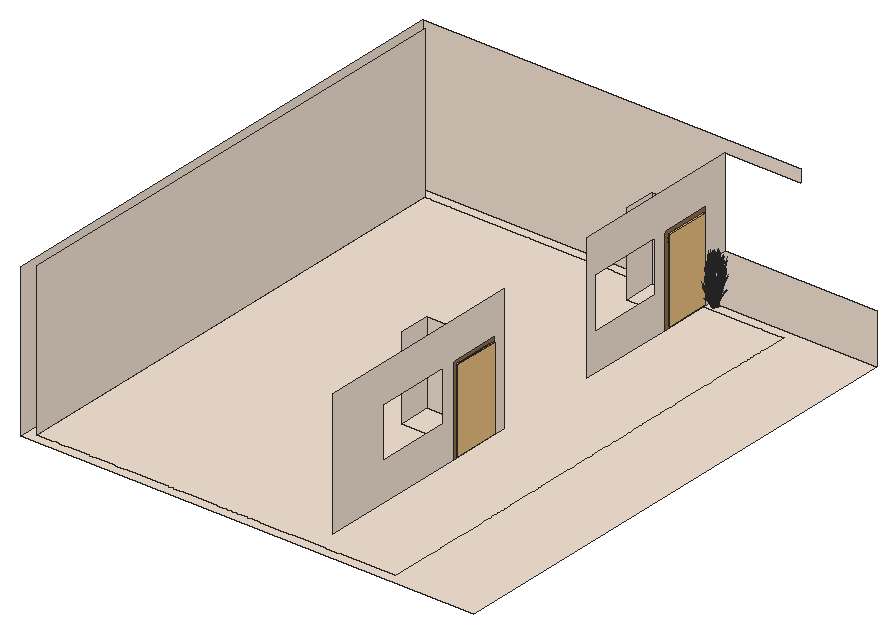
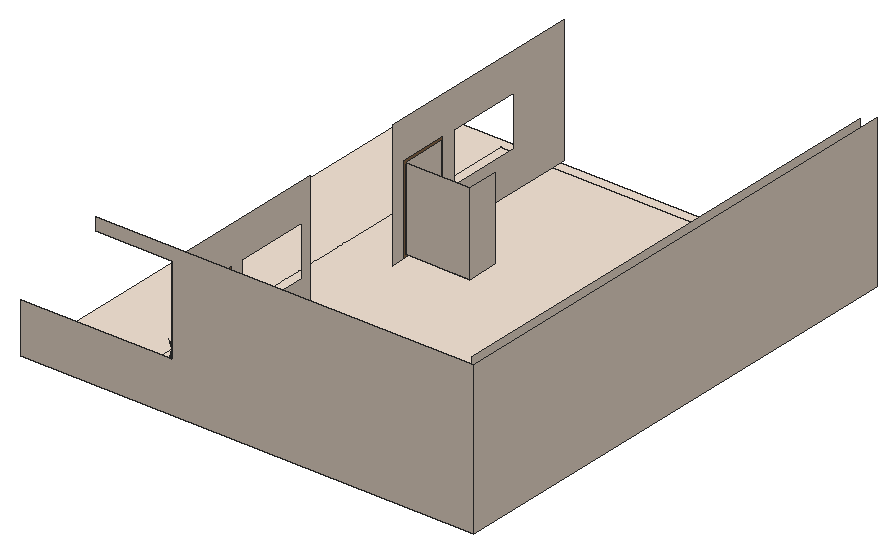
# SketchUp Ruby script. Lengths in inches.
U = 1.inch
M = Sketchup.active_model
def pt(a) = Geom::Point3d.new(a.map { |v| v * U })
def face(e, loops, mat)
  f = e.add_face(loops[0].map { |a| pt(a) })
  loops[1..].each { |l| e.add_face(l.map { |a| pt(a) }).erase! }
  f.material = f.back_material = mat if mat
  f
end
# faces: each face lists its corners as indices into pts; further lists are holes
def faces(e, pts, list, mat = nil) = list.each { |f| face(e, (f[0].is_a?(Array) ? f : [f]).map { |l| l.map { |i| pts[i] } }, mat) }
# xy, xz, yz: faces in a plane at the given z, y or x. An outline is a flat list of corners, or four numbers for a rectangle; further outlines are holes
def ring(l) = l.size == 4 ? [[l[0], l[1]], [l[2], l[1]], [l[2], l[3]], [l[0], l[3]]] : l.each_slice(2).to_a
def flat(e, list, mat, &to3) = list.each { |f| face(e, (f[0].is_a?(Array) ? f : [f]).map { |l| ring(l).map { |u, v| to3.(u, v) } }, mat) }
def xy(e, z, list, mat = nil) = flat(e, list, mat) { |x, y| [x, y, z] }
def xz(e, y, list, mat = nil) = flat(e, list, mat) { |x, z| [x, y, z] }
def yz(e, x, list, mat = nil) = flat(e, list, mat) { |y, z| [x, y, z] }
def lines(e, pts, list) = list.each { |a, b| e.add_line(pt(pts[a]), pt(pts[b])) }
# prism: a flat outline (further loops are holes) pulled along v
def prism(e, loops, v, mat = nil)
  f = face(e, loops, mat); d = Geom::Vector3d.new(v.map { |x| x * U })
  f.pushpull(f.normal.samedirection?(d) ? d.length : -d.length)
end
def box(e, o, s, mat = nil) = prism(e, [[o, [o[0] + s[0], o[1], o[2]], [o[0] + s[0], o[1] + s[1], o[2]], [o[0], o[1] + s[1], o[2]]]], [0, 0, s[2]], mat)
def at(x, y, z, deg = 0) = Geom::Transformation.translation(pt([x, y, z])) * Geom::Transformation.rotation(ORIGIN, Z_AXIS, deg.degrees)
def axes(o, x, y, z) = Geom::Transformation.new([*x, 0, *y, 0, *z, 0, *pt(o).to_a, 1])
def part(name) = M.definitions.add(name)
# library, detail: a bought-in or finely detailed component or shape, given as its bounding box
def library(name, o, s) = part(name).tap { |d| box(d.entities, o, s) }
def detail(e, o, s) = box(e.add_group.entities, o, s)
def put(e, d, t, mat = nil) = e.add_instance(d, t).tap { |i| i.material = mat if mat }
def group(e, t, mat = nil) = e.add_group.tap { |g| g.transformation = t; g.material = mat if mat }.entities
root = M.entities
M.materials.add("C01_Vanilla_Cream").color = [244, 228, 212]
M.materials.add("LightPink_Translucent").color = [144, 107, 117]
M.materials["LightPink_Translucent"].alpha = 0.75
M.materials.add("Wood_Floor_01_1K").color = [146, 111, 76]
c1 = part("blade")
p = [[2.15,0.21,22],[0,0.17,0],[0.09,0.45,0],[2.18,0.31,22],[2.29,0.31,22],[0.38,0.45,0],
  [2.48,0.24,33],[2.49,0.24,33],[2.48,0.22,33]]
faces(c1.entities,p,[[0,1,2,3],[4,5,2,3],[6,3,4,7],[8,0,3,6]])
c2 = part("seeds")
p = [[0.3,-0.1,1.38],[-0.01,-0.03,1.59],[-0.01,-0.03,0.03],[0.14,-0.07,-0.07],[0.29,-0.03,3],[0.15,0.01,3.11]]
faces(c2.entities,p,[[0,1,2,3],[1,0,4,5]],"LightPink_Translucent")
c3 = part("blade with seeds")
put(c3.entities,c1,at(0,0,0))
put(c3.entities,c2,axes([2.4,0.25,30.99],[1.5799,-0.05474,1.17369],[-0.12525,1.92788,0.29478],[-0.07173,-0.02425,1.56792]))
c4 = library("porta+4",[0.2,-5.42,1.33],[46.55,4.72,83.21])
xy(root,0,[[[0,0,432,480],[9,9,351,471]],[9,9,351,471]],"C01_Vanilla_Cream")
xy(root,15,[[226.53,171,288,201],[240,423,288,453]],"C01_Vanilla_Cream")
xz(root,201,[[226.53,15,288,93]],"C01_Vanilla_Cream")
xz(root,453,[[240,15,288,93]],"C01_Vanilla_Cream")
xz(root,480,[[0,0,0,144,360,144,360,132,288,132,288,48,432,48,432,0]],"C01_Vanilla_Cream")
yz(root,0,[[0,0,480,144]],"C01_Vanilla_Cream")
yz(root,9,[[9,0,471,144]],"C01_Vanilla_Cream")
yz(root,226.53,[[171,15,201,93]],"C01_Vanilla_Cream")
yz(root,240,[[423,15,453,93]],"C01_Vanilla_Cream")
yz(root,288,[[[12,12,156,12,156,96,204,96,204,12,216,12,216,132,12,132],[72,48,144,96]],[[314.71,12,408,12,408,96,456,96,456,12,468,12,468,48,480,48,480,132,314.71,132],[324,48,396,96]],[159,15,201,93],[411,15,453,93]],"C01_Vanilla_Cream")
yz(root,288,[[[156,12,204,96],[159,15,201,93]],[[408,12,456,96],[411,15,453,93]]],"Wood_Floor_01_1K")
put(root,c3,axes([294,457.43,14.91],[0.23093,-0.01116,1.28532],[-0.15319,0.4836,0.10393],[-0.32909,-0.02991,0.54946]))
put(root,c3,axes([294.1,458.28,14.91],[0.19317,-0.10421,1.28532],[0.16263,0.48153,0.10393],[-0.30326,0.10883,0.54946]))
put(root,c3,axes([293.5,459.1,13.94],[0.19348,0.04044,1.07251],[0.1247,0.41309,-0.23066],[-0.26282,0.07733,0.45856]))
put(root,c3,axes([295.21,457.78,14.51],[0.15825,-0.07127,1.32798],[0.05457,0.4976,0.10393],[-0.34278,0.06603,0.47463]))
put(root,c4,axes([291.16,410.82,13.74],[0,0.8978,0],[0.58403,0,0],[0,0,0.94]),"C01_Vanilla_Cream")
put(root,c3,axes([293.51,458.11,15.54],[-0.09091,0.06396,1.31208],[0.00773,0.46734,-0.2075],[-0.20839,0.06078,0.10523]))
put(root,c3,axes([294.69,456.98,15.74],[-0.55654,-0.01186,-0.53284],[0.03738,-0.49951,0.0643],[-0.23578,-0.05271,0.75375]))
put(root,c3,axes([294.25,457.1,13.94],[0.1087,0.13716,1.07251],[-0.25048,0.37284,-0.23066],[-0.25719,-0.08912,0.45856]))
put(root,c3,axes([293.8,457.84,15.39],[-0.46269,-0.13744,-0.2656],[0.13495,-0.40096,0.3429],[-0.18628,0.03677,0.65611]))
put(root,c3,axes([294.44,456.65,14.91],[0.2068,0.08488,1.28532],[-0.42797,0.35609,0.10393],[-0.26673,-0.16064,0.54946]))
put(root,c3,axes([292.5,458.58,15.53],[0.07105,0.01321,1.33037],[0.2198,0.43529,-0.12571],[-0.14545,0.11425,0.23543]))
put(root,c3,axes([294.12,458.05,15.51],[-0.15083,0.44814,-0.38324],[-0.51712,-0.15361,-0.29685],[-0.2082,0.04109,0.7333]))
put(root,c3,axes([294.51,457.08,15.51],[-0.40426,0.32635,-0.38324],[-0.35404,-0.34474,-0.29685],[-0.2054,-0.04965,0.7333]))
put(root,c3,axes([293.86,458.02,13.12],[0.01412,0.07764,1.32257],[-0.28464,0.40547,-0.20205],[-0.20218,-0.02044,0.22528]))
put(root,c3,axes([293.9375,456.17,15.53],[0.04127,0.04917,1.33037],[-0.19898,0.44196,-0.12571],[-0.20151,0.0032,0.23543]))
put(root,c3,axes([293.09,459.97,14.07],[0.23202,-0.22328,0.86145],[0.09155,0.35348,0.63294],[-0.16768,0.06329,0.18974]))
put(root,c3,axes([294.4,455.87,15.54],[-0.11979,-0.00348,1.31208],[-0.38137,0.34775,-0.2075],[-0.20349,-0.07106,0.10523]))
put(root,c3,axes([293.91,457.79,15.55],[0.15729,-0.44921,0.36002],[0.51712,0.15361,0.29685],[-0.20336,0.027,0.74497]))
put(root,c4,axes([289.83,157.29,13.73],[0,0.9504,0],[-0.24166,0,0],[0,0,0.9416]),"C01_Vanilla_Cream")
put(root,c3,axes([294.09,457.67,15.78],[0.28012,0.44611,-0.0912],[-0.49717,0.21923,-0.50621],[-0.20951,0.05886,0.76918]))
put(root,c3,axes([294.72,456.74,15.78],[-0.02981,0.50103,-0.0912],[-0.56442,-0.01369,-0.50621],[-0.21738,-0.0348,0.76918]))
put(root,c3,axes([294.36,456.77,15.39],[-0.31678,-0.30846,-0.2656],[0.36171,-0.29199,0.3429],[-0.18378,-0.04443,0.65611]))
put(root,c3,axes([293.87,457.68,15.55],[-0.20448,-0.33592,0.04823],[0.37288,-0.16442,0.37966],[-0.16437,0.03244,0.57892]))
put(root,c3,axes([294.81,458.6,14.91],[0.13906,-0.15138,1.28532],[0.35111,0.40859,0.10393],[-0.24082,0.18608,0.54946]))
put(root,c3,axes([293.97,459,15.39],[-0.48462,0.07041,-0.2656],[-0.12797,-0.4025,0.3429],[-0.13888,0.10811,0.65611]))
put(root,c3,axes([293.71,460.2,13.12],[0.07468,0.04922,1.32257],[0.12663,0.45605,-0.20205],[-0.16551,0.09725,0.22528]))
put(root,c3,axes([293.6,457.51,14.07],[0.35544,-0.03525,0.86145],[-0.22547,0.31061,0.63294],[-0.17565,-0.04659,0.18974]))
put(root,c3,axes([294.03,458.91,15.55],[-0.13808,-0.45342,0.36002],[0.54163,-0.07869,0.29685],[-0.15963,0.10664,0.74497]))
put(root,c3,axes([294.3125,456.66,15.82],[0.45978,-0.36358,0.40322],[0.39653,0.38611,0.33247],[-0.21571,-0.06707,0.83437]))
put(root,c3,axes([293.93,458.83,15.55],[-0.3822,-0.20719,0.04823],[0.22252,-0.29505,0.37966],[-0.12254,0.09539,0.57892]))
put(root,c3,axes([294.7,458.98,14.91],[0.10366,-0.16934,1.28532],[0.43488,0.35044,0.10393],[-0.19618,0.21841,0.54946]))
put(root,c3,axes([294.29,457.8,15.79],[0.46269,0.13744,0.2656],[-0.13495,0.40096,-0.3429],[-0.18628,0.03677,0.65611]))
put(root,c3,axes([294.37,459.05,15.51],[0.14302,0.44985,-0.38324],[-0.54163,0.07869,-0.29685],[-0.15522,0.12083,0.7333]))
put(root,c3,axes([294.52,456.66,15.55],[0.02803,-0.37463,0.04823],[0.42332,0.01027,0.37966],[-0.16216,-0.0392,0.57892]))
put(root,c3,axes([293.52,459.86,15.54],[-0.01384,0.09749,1.31208],[0.39274,0.33916,-0.2075],[-0.10282,0.16039,0.10523]))
put(root,c3,axes([295.72,458.72,13.54],[-0.57914,-0.08077,-0.46765],[0.12221,-0.49823,-0.12274],[-0.17283,-0.06037,1.03225]))
put(root,c3,axes([295.82,456.01,16.07],[-0.37157,0.4723,-0.10215],[-0.5381,-0.2721,-0.56695],[-0.18705,-0.13344,0.86148]))
put(root,c3,axes([294.81,456.93,15.79],[0.31678,0.30846,0.2656],[-0.36171,0.29199,-0.3429],[-0.18378,-0.04443,0.65611]))
put(root,c3,axes([295.66,456.39,15.74],[-0.47473,-0.23813,-0.53284],[0.33738,-0.41728,0.0643],[-0.172,-0.14218,0.75375]))
put(root,c3,axes([295.44,456.4,15.51],[-0.54938,0.11711,-0.38324],[-0.0961,-0.44351,-0.29685],[-0.14756,-0.1271,0.7333]))
put(root,c3,axes([294.96,459.67,13.51],[-0.52105,-0.24633,-0.37238],[0.31144,-0.44171,0],[-0.11867,-0.0561,1.18128]))
put(root,c3,axes([294.73,456,13.12],[-0.05393,0.0649,1.32257],[-0.545,0.13993,-0.20205],[-0.13166,-0.12729,0.22528]))
put(root,c3,axes([294.11,458.73,15.78],[0.515,0.27165,-0.0912],[-0.2967,0.3934,-0.50621],[-0.1455,0.13675,0.76918]))
put(root,c3,axes([295.28,459.97,13.78],[-0.34808,0.49367,0],[-0.58235,-0.27531,-0.38706],[-0.13264,-0.0627,1.22783]))
put(root,c3,axes([293.27,459.91,16.23],[0.49129,0.13151,-0.04866],[-0.15113,0.40475,-0.22062],[-0.08035,0.06145,0.72768]))
put(root,c3,axes([294.37,458.76,15.79],[0.48462,-0.07041,0.2656],[0.12797,0.4025,-0.3429],[-0.13888,0.10811,0.65611]))
put(root,c3,axes([294.64,460.68,13.94],[0.17569,-0.07772,1.07251],[0.43377,0.23434,-0.23066],[-0.12911,0.20277,0.45856]))
put(root,c3,axes([294.39,456.25,13.6],[-0.1606,0.40228,-0.02919],[-0.4943,-0.12375,-0.13237],[-0.07505,-0.0658,0.43661]))
put(root,c3,axes([295.68,454.88,15.53],[-0.01039,0.05905,1.33037],[-0.51226,0.21431,-0.12571],[-0.15074,-0.10955,0.23543]))
put(root,c3,axes([295.13,455.74,13.94],[-0.03371,0.16116,1.07251],[-0.49286,0.13491,-0.23066],[-0.11521,-0.20831,0.45856]))
put(root,c3,axes([295.29,456.16,14.91],[0.12726,0.15818,1.28532],[-0.58807,0.13317,0.10393],[-0.13291,-0.24832,0.54946]))
put(root,c3,axes([296.38,458.8,14],[-0.56211,0.32708,-0.21822],[-0.3738,-0.46216,-0.37502],[-0.13869,-0.04694,1.19781]))
put(root,c3,axes([294.82,459.83,15.55],[-0.39645,-0.33614,0.36002],[0.42102,-0.2899,0.29685],[-0.07313,0.15771,0.74497]))
put(root,c3,axes([295.5,456.08,15.39],[-0.08599,-0.39682,-0.2656],[0.49155,-0.10478,0.3429],[-0.13203,-0.11372,0.65611]))
put(root,c3,axes([294.13,458.08,13.78],[-0.69617,0,0],[0,-0.55062,-0.38706],[0,-0.12541,1.22783]))
put(root,c3,axes([295.11,459.48,13.52],[-0.13078,-0.42928,-0.23233],[0.51941,-0.1219,0.23233],[-0.10471,-0.0495,1.0423]))
put(root,c3,axes([294.68,459.8,15.55],[-0.45752,-0.02296,0.04823],[0.01254,-0.34663,0.37966],[-0.04787,0.13278,0.57892]))
put(root,c3,axes([294.82,459.93,15.39],[-0.3767,0.25939,-0.2656],[-0.3566,-0.29618,0.3429],[-0.05426,0.15048,0.65611]))
put(root,c3,axes([296.75,459.16,13.54],[-0.375,0.3703,-0.46765],[-0.46584,-0.33578,-0.12274],[-0.15027,0.09237,1.03225]))
put(root,c3,axes([295.79,456.4,15.79],[0.08599,0.39682,0.2656],[-0.49155,0.10478,-0.3429],[-0.13203,-0.11372,0.65611]))
put(root,c3,axes([293.48,460.86,15.53],[0.06316,-0.02974,1.33037],[0.52204,0.19785,-0.12571],[-0.01227,0.16473,0.23543]))
put(root,c3,axes([294.67,457.94,13.75],[-0.51786,0.4142,0.23067],[-0.51817,-0.40984,-0.27369],[-0.01808,-0.11762,1.23664]))
put(root,c3,axes([296.8,459.08,14.49],[0.48111,0.19866,1.13446],[-0.47133,0.42798,0.44862],[-0.21112,-0.25366,0.95105]))
put(root,c3,axes([294.96,455.48,14.07],[0.29042,0.17147,0.86145],[-0.42295,0.10307,0.63294],[-0.0905,-0.13178,0.18974]))
put(root,c3,axes([297.01,458.95,13.85],[-0.54364,-0.39653,-0.18894],[0.45745,-0.44527,0.41347],[-0.14639,0.04639,1.26162]))
put(root,c3,axes([296.02,458.57,13.66],[-0.33445,-0.41351,-0.33554],[0.50659,-0.29119,0.16149],[-0.10823,-0.05117,1.07733]))
put(root,c3,axes([295.07,459.66,16],[-0.01449,0.45571,-0.59145],[-0.61002,-0.03061,0.07138],[-0.06438,0.19306,0.83667]))
put(root,c3,axes([295.0625,460.94,14.07],[-0.01441,-0.29294,0.86145],[0.36003,0.20894,0.63294],[-0.07081,0.13963,0.18974]))
put(root,c3,axes([295.57,455.93,15.82],[0.62019,-0.12663,0.40322],[0.10763,0.49673,0.33247],[-0.14586,-0.1464,0.83437]))
put(root,c3,axes([296.73,458.86,13.66],[-0.60457,0.03041,-0.33554],[-0.05467,-0.50484,0.16149],[-0.10823,0.05117,1.07733]))
put(root,c3,axes([295.71,456.04,15.55],[0.25304,-0.31296,0.04823],[0.36033,0.18221,0.37966],[-0.11649,-0.10034,0.57892]))
put(root,c3,axes([295.58,459.71,13.86],[0.52105,0.24633,0.37238],[-0.31144,0.44171,0],[-0.11867,-0.0561,1.18128]))
put(root,c3,axes([294.87,460.3,14.52],[0.01223,-0.25433,1.15759],[0.55017,0.13434,0.15997],[-0.04767,0.27105,0.54661]))
put(root,c3,axes([296.07,458.8,13.83],[0.14756,-0.58378,-0.17572],[0.69966,0.10176,0.38453],[-0.12225,-0.08062,1.1733]))
put(root,c3,axes([296.32,458.94,13.96],[-0.1074,0.43968,0.1086],[-0.52474,-0.07632,-0.3101],[-0.0955,-0.04515,0.95058]))
put(root,c3,axes([296.26,455.11,15.54],[-0.08515,-0.06907,1.31208],[-0.56828,0.04379,-0.2075],[-0.0907,-0.16522,0.10523]))
put(root,c3,axes([297.37,460.17,13.51],[-0.52105,0.24633,-0.37238],[-0.31144,-0.44171,0],[-0.11867,0.0561,1.18128]))
put(root,c3,axes([294.28,457.71,13.51],[0,-0.49266,-0.37238],[0.62289,0,0],[0,-0.11221,1.18128]))
put(root,c3,axes([294.55,458.17,13.86],[0,0.49266,0.37238],[-0.62289,0,0],[0,-0.11221,1.18128]))
put(root,c3,axes([297.4,460.03,13.64],[-0.34375,-0.4954,-0.03857],[0.58235,-0.27531,0.38706],[-0.1435,0.04717,1.22723]))
put(root,c3,axes([295.2,459.81,15.75],[0.39855,0.33102,-0.4254],[-0.42102,0.2899,-0.32951],[-0.06064,0.16819,0.81396]))
put(root,c3,axes([297.25,459.97,13.52],[-0.51941,-0.1219,-0.23233],[0.13078,-0.42928,0.23233],[-0.10471,0.0495,1.0423]))
put(root,c3,axes([295.02,459.5625,15.79],[0.3767,-0.25939,0.2656],[0.3566,0.29618,-0.3429],[-0.05426,0.15048,0.65611]))
put(root,c3,axes([295.91,458.28,14],[-0.62699,-0.23507,-0.21822],[0.3019,-0.49615,-0.37502],[-0.0197,-0.12182,1.19781]))
put(root,c3,axes([297.54,458.14,14.13],[-0.01521,-0.46386,1.05954],[0.68831,0.12024,0.44862],[-0.1628,0.25382,1.00012]))
put(root,c3,axes([294.78,459.64,16.05],[0.61188,0.02441,-0.10123],[-0.01672,0.46217,-0.56189],[-0.0425,0.178,0.85379]))
put(root,c3,axes([294.76,460.31,14.12],[0.50577,-0.08724,0.04881],[0.11627,0.35148,-0.64728],[-0.03206,0.17792,0.5802]))
put(root,c3,axes([297.16,458.73,14],[0.06488,0.56215,-0.21822],[-0.6757,0.03399,-0.37502],[-0.11898,0.07488,1.19781]))
put(root,c3,axes([295.63,457.78,13.57],[-0.22864,-0.5052,-0.52377],[0.65862,-0.18195,-0.13747],[-0.02527,-0.17107,1.15612]))
put(root,c3,axes([297.13,456.18,15.78],[-0.54481,0.22937,-0.0912],[-0.26773,-0.4071,-0.50621],[-0.07188,-0.17155,0.76918]))
put(root,c3,axes([296.66,456.2,15.51],[-0.54728,-0.1235,-0.38324],[0.18759,-0.42344,-0.29685],[-0.05018,-0.17048,0.7333]))
put(root,c3,axes([295.65,459.33,14.91],[-0.01363,-0.18909,1.28532],[0.5906,0.12544,0.10393],[-0.03653,0.26947,0.54946]))
put(root,c3,axes([294.55,457.72,13.52],[0.38863,-0.30738,-0.23233],[0.38863,0.30738,0.23233],[0,-0.09901,1.0423]))
put(root,c3,axes([296.31,455.73,13.6],[-0.38473,0.28263,-0.02919],[-0.35252,-0.30954,-0.13237],[-0.02482,-0.08771,0.43661]))
put(root,c3,axes([296.15,458.52,13.77],[0.70367,0.1038,0.34316],[-0.1432,0.58624,0.13466],[-0.10283,-0.05661,1.19142]))
put(root,c3,axes([295.97,458.42,14.04],[-0.27012,0.44393,0.33554],[-0.56127,-0.21365,-0.16149],[0,-0.10233,1.07733]))
put(root,c3,axes([296.86,456.28,15.74],[-0.26572,-0.40059,-0.53284],[0.54698,-0.22325,0.0643],[-0.06214,-0.19355,0.75375]))
put(root,c3,axes([295.77,459.46,13.86],[0.59825,-0.13076,0.13232],[0.14773,0.48663,0.26315],[-0.05336,-0.0709,1.20305]))
put(root,c3,axes([296.54,459.54,13.65],[-0.56127,-0.22118,0],[0.27012,-0.45959,0],[0,0,1.2203]))
put(root,c3,axes([296.96,456.34,15.79],[-0.16784,0.37886,0.2656],[-0.48968,-0.1105,-0.3429],[-0.0449,-0.15254,0.65611]))
put(root,c3,axes([297.84,460.09,13.78],[0.34808,0.49367,0],[-0.58235,0.27531,-0.38706],[-0.13264,0.0627,1.22783]))
put(root,c3,axes([296.07,460.3,15.8],[-0.54859,-0.1288,0.39962],[0.18759,-0.42344,0.32951],[0.03297,0.16652,0.82692]))
put(root,c3,axes([295.92,460.33,15.55],[-0.41024,0.16744,0.04823],[-0.2008,-0.30532,0.37966],[0.03962,0.13459,0.57892]))
put(root,c3,axes([297.55,459.49,13.86],[0.16083,-0.48962,0.13232],[0.58854,0.13856,0.26315],[-0.10167,0.00238,1.20305]))
put(root,c3,axes([297.28,458.84,13.96],[0.41131,0.296,0.1086],[-0.34309,0.33395,-0.3101],[-0.0955,0.04515,0.95058]))
put(root,c3,axes([297.13,458.47,13.72],[-0.51786,-0.42404,-0.04598],[0.51817,-0.4243,0],[-0.01808,-0.01481,1.31678]))
put(root,c3,axes([297.27,458.62,14.04],[0.60457,-0.03041,0.33554],[0.05467,0.50484,-0.16149],[-0.10823,0.05117,1.07733]))
put(root,c3,axes([297.42,459.78,13.75],[0.697,0.16013,0.23067],[-0.17437,0.57237,-0.27369],[-0.11536,0.07164,1.23664]))
put(root,c3,axes([296.4,455.39,13.12],[-0.09338,0.01775,1.32257],[-0.51641,-0.1998,-0.20205],[0.00867,-0.16666,0.22528]))
put(root,c3,axes([297.72,459.75,13.86],[0.52105,-0.24633,0.37238],[0.31144,0.44171,0],[-0.11867,0.0561,1.18128]))
put(root,c3,axes([296.91,455.9375,15.39],[0.16784,-0.37886,-0.2656],[0.48968,0.1105,0.3429],[-0.0449,-0.15254,0.65611]))
put(root,c3,axes([296.09,457.98,13.77],[0.24206,0.5509,0.34316],[-0.69162,0.19157,0.13466],[0.00845,-0.10123,1.19142]))
put(root,c3,axes([295.98,457.91,13.66],[0.27012,-0.44393,-0.33554],[0.56127,0.21365,0.16149],[0,-0.10233,1.07733]))
put(root,c3,axes([296.67,459.34,13.65],[-0.18165,-0.42474,0],[0.51872,-0.14874,0],[0,0,1.15778]))
put(root,c3,axes([296.01,460.24,13.12],[0.0901,-0.02681,1.32257],[0.54199,0.14755,-0.20205],[0.01585,0.1663,0.22528]))
put(root,c3,axes([296.13,460.39,15.39],[-0.16784,0.37886,-0.2656],[-0.48968,-0.1105,0.3429],[0.0449,0.15254,0.65611]))
put(root,c3,axes([297.4,458.51,13.66],[-0.27012,0.44393,-0.33554],[-0.56127,-0.21365,0.16149],[0,0.10233,1.07733]))
put(root,c3,axes([297.12,455.99,15.55],[0.41024,-0.16744,0.04823],[0.2008,0.30532,0.37966],[-0.03962,-0.13459,0.57892]))
put(root,c3,axes([295.78,461.0625,15.54],[0.07057,0.07933,1.31208],[0.56952,0.03117,-0.2075],[0.05727,0.17496,0.10523]))
put(root,c3,axes([298.47,458.24,13.86],[-0.43742,-0.35886,0.13232],[0.44081,-0.34807,0.26315],[-0.04831,0.07329,1.20305]))
put(root,c3,axes([296.96,458.03,13.65],[0,-0.57005,0],[0.69617,0,0],[0,0,1.34592]))
put(root,c3,axes([296.97,456.02,15.55],[0.54859,0.1288,0.36002],[-0.18759,0.42344,0.29685],[-0.03297,-0.16652,0.74497]))
put(root,c3,axes([296.3125,458.13,13.82],[0.6273,0.23878,0.18048],[-0.3019,0.49615,0.37502],[0,-0.11437,1.20407]))
put(root,c3,axes([297.31,458.26,13.72],[0,0.56976,-0.04228],[-0.69617,0,0],[0,0.01791,1.34526]))
put(root,c3,axes([296.11,457.8,14.04],[-0.60457,0.03041,0.33554],[-0.05467,-0.50484,-0.16149],[0.10823,-0.05117,1.07733]))
put(root,c3,axes([296.08,459.99,15.79],[0.16784,-0.37886,0.2656],[0.48968,0.1105,-0.3429],[0.0449,0.15254,0.65611]))
put(root,c3,axes([295.83,456.93,13.86],[-0.16083,0.48962,0.13232],[-0.58854,-0.13856,0.26315],[0.10167,-0.00238,1.20305]))
put(root,c3,axes([296.98,459.36,13.72],[0.24206,0.56598,-0.04509],[-0.69162,0.19832,0],[0.00845,0.01976,1.2913]))
put(root,c3,axes([295.54,456.33,13.78],[-0.34808,-0.49367,0],[0.58235,-0.27531,-0.38706],[0.13264,-0.0627,1.22783]))
put(root,c3,axes([296.18,460.05,15.74],[0.26572,0.40059,-0.53284],[-0.54698,0.22325,0.0643],[0.06214,0.19355,0.75375]))
put(root,c3,axes([298.98,458.62,13.65],[-0.69582,-0.00394,-0.03732],[0,-0.55062,0.37457],[-0.02187,0.12535,1.18764]))
put(root,c3,axes([297.61,456.96,13.86],[-0.59825,0.13076,0.13232],[-0.14773,-0.48663,0.26315],[0.05336,0.0709,1.20305]))
put(root,c3,axes([297,455.14,14.07],[0.07142,0.28728,0.86145],[-0.3962,-0.15911,0.63294],[0.04263,-0.1471,0.18974]))
put(root,c3,axes([296.73,461.34,16.23],[0.38473,-0.28263,-0.04866],[0.35252,0.30954,-0.22062],[0.02482,0.08771,0.72768]))
put(root,c3,axes([296.63,457.67,13.77],[-0.46162,0.4471,0.34316],[-0.54842,-0.39467,0.13466],[0.11129,-0.04462,1.19142]))
put(root,c3,axes([297.42,458.375,13.66],[0.38863,0.31822,0],[-0.38863,0.31822,0],[0,0,1.2695]))
put(root,c3,axes([297.41,458,14.04],[0.27012,-0.44393,0.33554],[0.56127,0.21365,-0.16149],[0,0.10233,1.07733]))
put(root,c3,axes([297.18,459.54,13.65],[0.56127,0.22118,0],[-0.27012,0.45959,0],[0,0,1.31215]))
put(root,c3,axes([296.38,460.13,15.51],[0.54728,0.1235,-0.38324],[-0.18759,0.42344,-0.29685],[0.05018,0.17048,0.7333]))
put(root,c3,axes([295.91,460.15,15.78],[0.54481,-0.22937,-0.0912],[0.26773,0.4071,-0.50621],[0.07188,0.17155,0.76918]))
put(root,c3,axes([297.23,457.9,13.79],[-0.70367,-0.1038,0.36899],[0.1432,-0.58624,0.1448],[0.10283,0.05661,1.2811]))
put(root,c3,axes([298.7,455.61,15.53],[-0.05654,0.03763,1.33037],[-0.55396,-0.12696,-0.12571],[-0.02005,-0.16422,0.23543]))
put(root,c3,axes([298.26,456.69,15.78],[-0.61188,-0.02441,-0.0912],[0.01672,-0.46217,-0.50621],[0.0425,-0.178,0.76918]))
put(root,c3,axes([298.83,458.7,13.52],[-0.38863,0.30738,-0.23233],[-0.38863,-0.30738,0.23233],[0,0.09901,1.0423]))
put(root,c3,axes([297.72,458.64,13.57],[0.20414,0.45107,-0.51909],[-0.58805,0.16245,-0.13624],[0.02256,0.15274,1.1458]))
put(root,c3,axes([297.43,458.16,13.65],[0.62289,0,0],[0,0.51004,0],[0,0,1.33805]))
put(root,c3,axes([298.02,456.76,15.79],[-0.3767,0.25939,0.2656],[-0.3566,-0.29618,-0.3429],[0.05426,-0.15048,0.65611]))
put(root,c3,axes([296.83,457.59,14.04],[-0.33445,-0.41351,0.33554],[0.50659,-0.29119,-0.16149],[0.10823,0.05117,1.07733]))
put(root,c3,axes([296.22,457.69,14],[-0.06488,-0.56215,-0.21822],[0.6757,-0.03399,-0.37502],[0.11898,-0.07488,1.19781]))
put(root,c3,axes([297.65,458.1,13.96],[0.51872,-0.14368,0.1086],[0.18165,0.41027,-0.3101],[0,0.09029,0.95058]))
put(root,c3,axes([297.84,456.52,15.51],[-0.39855,-0.33102,-0.38324],[0.42102,-0.2899,-0.29685],[0.06064,-0.16819,0.7333]))
put(root,c3,axes([297.47,458.14,14],[0.62699,0.23507,-0.21822],[-0.3019,0.49615,-0.37502],[0.0197,0.12182,1.19781]))
put(root,c3,axes([296.14,456.45,13.52],[0.51941,0.1219,-0.23233],[-0.13078,0.42928,0.23233],[0.10471,-0.0495,1.0423]))
put(root,c3,axes([297.58,455.93,13.94],[-0.15825,0.09972,1.07251],[-0.47395,-0.17454,-0.23066],[0.08785,-0.21706,0.45856]))
put(root,c3,axes([298.83,458.25,13.86],[0,-0.49266,0.37238],[0.62289,0,0],[0,0.11221,1.18128]))
put(root,c3,axes([299.1,458.71,13.51],[0,0.49266,-0.37238],[-0.62289,0,0],[0,0.11221,1.18128]))
put(root,c3,axes([297.4375,460.2,15.55],[-0.55374,0.11306,0.36002],[-0.0961,-0.44351,0.29685],[0.13023,0.13071,0.74497]))
put(root,c3,axes([296.01,456.25,13.51],[0.52105,-0.24633,-0.37238],[0.31144,0.44171,0],[0.11867,-0.0561,1.18128]))
put(root,c3,axes([297.33,460.29,15.55],[-0.25304,0.31296,0.04823],[-0.36033,-0.18221,0.37966],[0.11649,0.10034,0.57892]))
put(root,c3,axes([296.69,459.26,14.91],[-0.12726,-0.15818,1.28532],[0.58807,-0.13317,0.10393],[0.13291,0.24832,0.54946]))
put(root,c3,axes([297.06,457.48,13.96],[0.1074,-0.43968,0.1086],[0.52474,0.07632,-0.3101],[0.0955,0.04515,0.95058]))
put(root,c3,axes([297.8,456.71,13.86],[-0.52105,-0.24633,0.37238],[0.31144,-0.44171,0],[0.11867,0.0561,1.18128]))
put(root,c3,axes([297.97,456.67,15.74],[0.01449,-0.45571,-0.53284],[0.61002,0.03061,0.0643],[0.06438,-0.19306,0.75375]))
put(root,c3,axes([297.35,459.28,13.64],[0.5845,-0.16716,-0.14398],[0.20539,0.48152,0.00006],[0.06452,-0.01848,1.30423]))
put(root,c3,axes([297.25,459.93,15.79],[-0.08599,-0.39682,0.2656],[0.49155,-0.10478,-0.3429],[0.13203,0.11372,0.65611]))
put(root,c3,axes([297.36,457.85,13.66],[0.33445,0.41351,-0.33554],[-0.50659,0.29119,0.16149],[0.10823,0.05117,1.07733]))
put(root,c3,axes([297.58,457.65,15.36],[-0.48108,-0.25598,1.03712],[0.50798,-0.39855,0.44749],[0.15521,0.24018,1.00248]))
put(root,c3,axes([298.22,456.39,15.39],[0.3767,-0.25939,-0.2656],[0.3566,0.29618,0.3429],[0.05426,-0.15048,0.65611]))
put(root,c3,axes([296.77,460.48,15.53],[0.00165,-0.05965,1.33037],[0.47711,-0.26315,-0.12571],[0.16572,0.09393,0.23543]))
